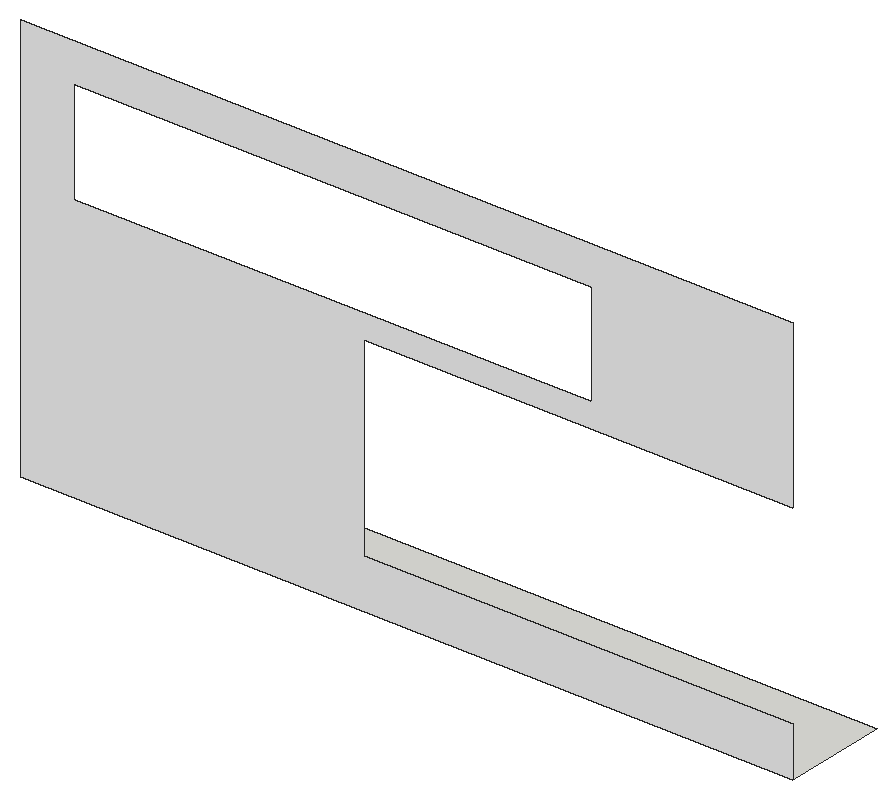
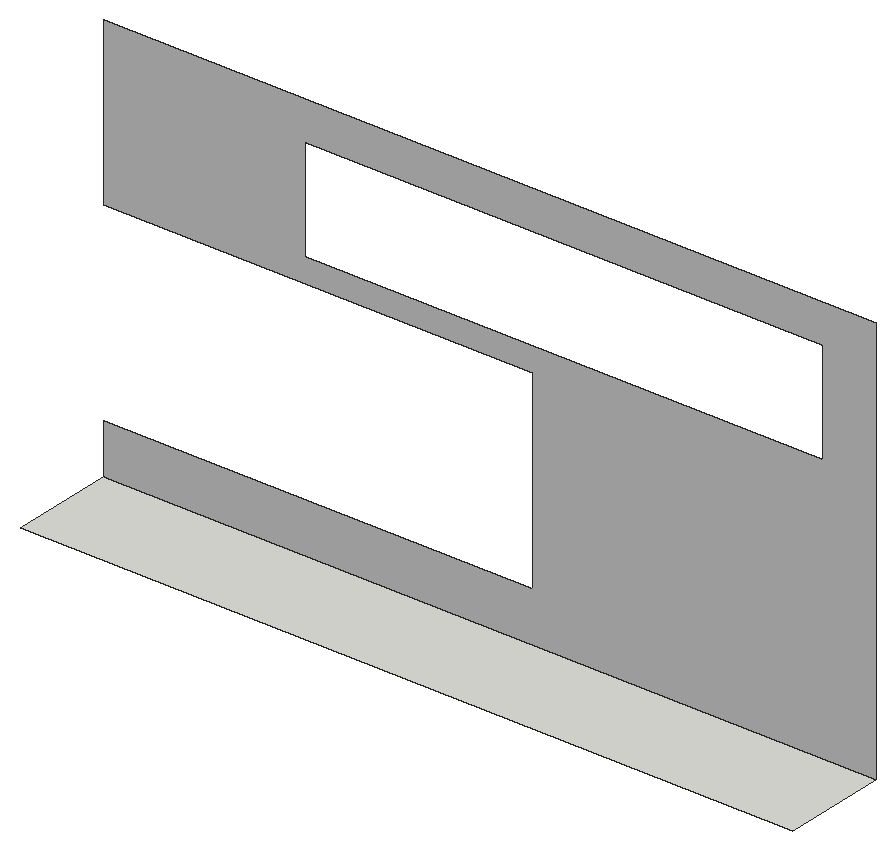
# SketchUp Ruby script. Lengths in inches.
U = 1.inch
M = Sketchup.active_model
def pt(a) = Geom::Point3d.new(a.map { |v| v * U })
def face(e, loops, mat)
  f = e.add_face(loops[0].map { |a| pt(a) })
  loops[1..].each { |l| e.add_face(l.map { |a| pt(a) }).erase! }
  f.material = f.back_material = mat if mat
  f
end
# faces: each face lists its corners as indices into pts; further lists are holes
def faces(e, pts, list, mat = nil) = list.each { |f| face(e, (f[0].is_a?(Array) ? f : [f]).map { |l| l.map { |i| pts[i] } }, mat) }
# xy, xz, yz: faces in a plane at the given z, y or x. An outline is a flat list of corners, or four numbers for a rectangle; further outlines are holes
def ring(l) = l.size == 4 ? [[l[0], l[1]], [l[2], l[1]], [l[2], l[3]], [l[0], l[3]]] : l.each_slice(2).to_a
def flat(e, list, mat, &to3) = list.each { |f| face(e, (f[0].is_a?(Array) ? f : [f]).map { |l| ring(l).map { |u, v| to3.(u, v) } }, mat) }
def xy(e, z, list, mat = nil) = flat(e, list, mat) { |x, y| [x, y, z] }
def xz(e, y, list, mat = nil) = flat(e, list, mat) { |x, z| [x, y, z] }
def yz(e, x, list, mat = nil) = flat(e, list, mat) { |y, z| [x, y, z] }
def lines(e, pts, list) = list.each { |a, b| e.add_line(pt(pts[a]), pt(pts[b])) }
# prism: a flat outline (further loops are holes) pulled along v
def prism(e, loops, v, mat = nil)
  f = face(e, loops, mat); d = Geom::Vector3d.new(v.map { |x| x * U })
  f.pushpull(f.normal.samedirection?(d) ? d.length : -d.length)
end
def box(e, o, s, mat = nil) = prism(e, [[o, [o[0] + s[0], o[1], o[2]], [o[0] + s[0], o[1] + s[1], o[2]], [o[0], o[1] + s[1], o[2]]]], [0, 0, s[2]], mat)
def at(x, y, z, deg = 0) = Geom::Transformation.translation(pt([x, y, z])) * Geom::Transformation.rotation(ORIGIN, Z_AXIS, deg.degrees)
def axes(o, x, y, z) = Geom::Transformation.new([*x, 0, *y, 0, *z, 0, *pt(o).to_a, 1])
def part(name) = M.definitions.add(name)
# library, detail: a bought-in or finely detailed component or shape, given as its bounding box
def library(name, o, s) = part(name).tap { |d| box(d.entities, o, s) }
def detail(e, o, s) = box(e.add_group.entities, o, s)
def put(e, d, t, mat = nil) = e.add_instance(d, t).tap { |i| i.material = mat if mat }
def group(e, t, mat = nil) = e.add_group.tap { |g| g.transformation = t; g.material = mat if mat }.entities
root = M.entities
M.materials.add("[Blinds Vertical Stripe Gray]1").color = [252, 252, 252]
xy(root,0,[[206.19,96.24,315.3,111]])
xz(root,96.24,[[[206.19,0,315.3,0,315.3,7.1,254.71,7.1,254.71,34.41,315.3,34.41,315.3,57.8125,206.19,57.8125],[213.78,37.78,286.85,52.34]]],"[Blinds Vertical Stripe Gray]1")
